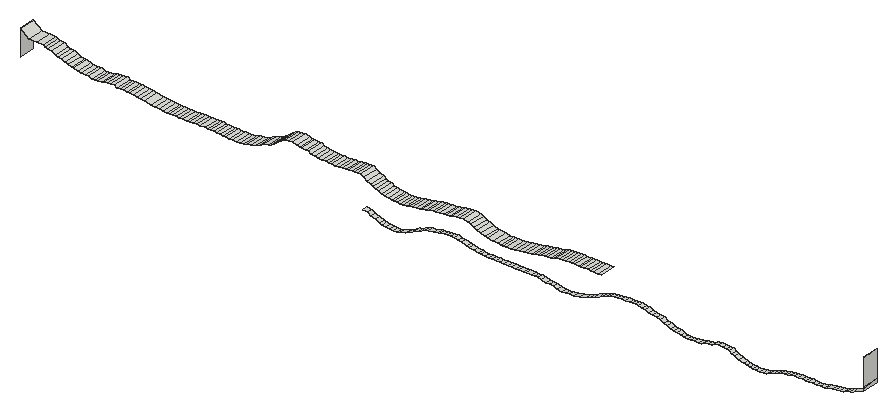
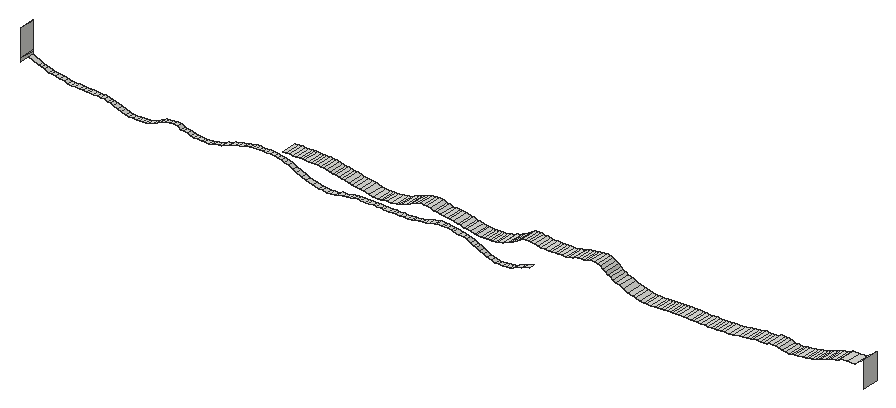
# SketchUp Ruby script. Lengths in inches.
U = 1.inch
M = Sketchup.active_model
def pt(a) = Geom::Point3d.new(a.map { |v| v * U })
def face(e, loops, mat)
  f = e.add_face(loops[0].map { |a| pt(a) })
  loops[1..].each { |l| e.add_face(l.map { |a| pt(a) }).erase! }
  f.material = f.back_material = mat if mat
  f
end
# faces: each face lists its corners as indices into pts; further lists are holes
def faces(e, pts, list, mat = nil) = list.each { |f| face(e, (f[0].is_a?(Array) ? f : [f]).map { |l| l.map { |i| pts[i] } }, mat) }
# xy, xz, yz: faces in a plane at the given z, y or x. An outline is a flat list of corners, or four numbers for a rectangle; further outlines are holes
def ring(l) = l.size == 4 ? [[l[0], l[1]], [l[2], l[1]], [l[2], l[3]], [l[0], l[3]]] : l.each_slice(2).to_a
def flat(e, list, mat, &to3) = list.each { |f| face(e, (f[0].is_a?(Array) ? f : [f]).map { |l| ring(l).map { |u, v| to3.(u, v) } }, mat) }
def xy(e, z, list, mat = nil) = flat(e, list, mat) { |x, y| [x, y, z] }
def xz(e, y, list, mat = nil) = flat(e, list, mat) { |x, z| [x, y, z] }
def yz(e, x, list, mat = nil) = flat(e, list, mat) { |y, z| [x, y, z] }
def lines(e, pts, list) = list.each { |a, b| e.add_line(pt(pts[a]), pt(pts[b])) }
# prism: a flat outline (further loops are holes) pulled along v
def prism(e, loops, v, mat = nil)
  f = face(e, loops, mat); d = Geom::Vector3d.new(v.map { |x| x * U })
  f.pushpull(f.normal.samedirection?(d) ? d.length : -d.length)
end
def box(e, o, s, mat = nil) = prism(e, [[o, [o[0] + s[0], o[1], o[2]], [o[0] + s[0], o[1] + s[1], o[2]], [o[0], o[1] + s[1], o[2]]]], [0, 0, s[2]], mat)
def at(x, y, z, deg = 0) = Geom::Transformation.translation(pt([x, y, z])) * Geom::Transformation.rotation(ORIGIN, Z_AXIS, deg.degrees)
def axes(o, x, y, z) = Geom::Transformation.new([*x, 0, *y, 0, *z, 0, *pt(o).to_a, 1])
def part(name) = M.definitions.add(name)
# library, detail: a bought-in or finely detailed component or shape, given as its bounding box
def library(name, o, s) = part(name).tap { |d| box(d.entities, o, s) }
def detail(e, o, s) = box(e.add_group.entities, o, s)
def put(e, d, t, mat = nil) = e.add_instance(d, t).tap { |i| i.material = mat if mat }
def group(e, t, mat = nil) = e.add_group.tap { |g| g.transformation = t; g.material = mat if mat }.entities
root = M.entities
xy(root,238.18,[[1254.78,2401.37,1255.46,2402.3]])
xy(root,238.62,[[1221.31,2401.37,1222.08,2402.3],[1222.08,2401.37,1222.71,2402.3],[1222.71,2401.37,1223.47,2402.3],[1223.47,2401.37,1224.09,2402.3],[1224.09,2401.37,1224.94,2402.3],
  [1224.94,2401.37,1225.58,2402.3],[1225.58,2401.37,1226.2,2402.3]])
xy(root,238.625,[[1219.89,2401.37,1220.75,2402.3]])
xy(root,238.89,[[1275.7,2401.37,1276.38,2402.3]])
xy(root,238.9,[[1277.14,2401.37,1277.76,2402.3],[1277.76,2401.37,1278.53,2402.3]])
xy(root,240.43,[[1243.98,2401.37,1244.55,2402.3]])
xy(root,241.68,[[1162.03,2401.37,1162.62,2404.3]])
xy(root,241.75,[[1164.38,2401.37,1165.25,2404.3],[1165.25,2401.37,1165.87,2404.3],[1165.87,2401.37,1166.38,2404.3]])
xy(root,243.05,[[1237.04,2401.37,1237.72,2404.3]])
xy(root,243.07,[[1235.1875,2401.37,1235.77,2404.3]])
xy(root,243.09,[[1231.875,2401.37,1232.4,2404.3],[1232.4,2401.37,1232.92,2404.3],[1232.92,2401.37,1233.58,2404.3],[1233.58,2401.37,1234.03,2404.3]])
yz(root,1131.59,[[2401.37,241.52,2404.3,246.2]])
yz(root,1285.6,[[2401.37,240.89,2401.37,241.29,2404.3,241.52,2404.3,240.89],[2401.37,241.29,2404.3,241.52,2401.37,241.52],[2401.37,241.52,2401.37,246.27,2402.0625,246.36,2404.3,246.43,2404.3,241.52],[2401.37,246.27,2401.37,246.43,2404.3,246.43,2402.0625,246.36]])
p = [[1198.39,2401.37,237.11],[1198.39,2402.3,237.11],[1199.15,2402.3,237.04],[1199.15,2401.37,237.04],[1199.84,2402.3,237.01],[1199.84,2401.37,237.01],
  [1200.45,2402.3,236.98],[1200.45,2401.37,236.98],[1201.13,2402.3,237.22],[1201.13,2401.37,237.22],[1197.7,2401.37,237.2],[1197.7,2402.3,237.2],
  [1197.17,2401.37,237.33],[1197.17,2402.3,237.33],[1201.98,2402.3,237.43],[1201.98,2401.37,237.43],[1196.5,2401.37,237.68],[1196.5,2402.3,237.68],
  [1202.6,2402.3,237.74],[1202.6,2401.37,237.74],[1265.43,2401.37,237.45],[1265.43,2402.3,237.45],[1266,2402.3,237.42],[1266,2401.37,237.42],
  [1266.73,2402.3,237.4],[1266.73,2401.37,237.4],[1267.41,2402.3,237.47],[1267.41,2401.37,237.47],[1264.24,2401.37,237.59],[1264.24,2402.3,237.59],
  [1264.84,2402.3,237.51],[1264.84,2401.37,237.51],[1268.01,2402.3,237.5625],[1268.01,2401.37,237.5625],[1263.7,2401.37,237.71],[1263.7,2402.3,237.71],
  [1268.7,2402.3,237.84],[1268.7,2401.37,237.84],[1195.5625,2401.37,237.96],[1195.5625,2402.3,237.96],[1203.3,2402.3,238.02],[1203.3,2401.37,238.02],
  [1230.44,2401.37,237.79],[1230.44,2402.3,237.79],[1231.15,2402.3,237.74],[1231.15,2401.37,237.74],[1232.02,2402.3,237.87],[1232.02,2401.37,237.87],
  [1262.87,2401.37,238],[1262.87,2402.3,238],[1229.67,2401.37,237.86],[1229.67,2402.3,237.86],[1269.38,2402.3,238.08],[1269.38,2401.37,238.08],
  [1229.04,2401.37,238.15],[1229.04,2402.3,238.15],[1232.67,2402.3,237.88],[1232.67,2401.37,237.88],[1233.79,2402.3,238.14],[1233.79,2401.37,238.14],
  [1195,2401.37,238.28],[1195,2402.3,238.28],[1203.74,2402.3,238.375],[1203.74,2401.37,238.375],[1262.16,2401.37,238.33],[1262.16,2402.3,238.33],
  [1228.27,2401.37,238.19],[1228.27,2402.3,238.19],[1235.01,2402.3,238.46],[1235.01,2401.37,238.46],[1252.76,2401.37,238.19],[1252.76,2402.3,238.19],
  [1253.58,2402.3,238.15],[1253.58,2401.37,238.15],[1254.11,2402.3,238.11],[1254.11,2401.37,238.11],[1254.78,2402.3,238.18],[1254.78,2401.37,238.18],
  [1270.07,2402.3,238.33],[1270.07,2401.37,238.33],[1227.65,2401.37,238.25],[1227.65,2402.3,238.25],[1252.1875,2401.37,238.26],[1252.1875,2402.3,238.26],
  [1255.46,2401.37,238.18],[1255.46,2402.3,238.18],[1256.14,2402.3,238.27],[1256.14,2401.37,238.27],[1194.22,2401.37,238.43],[1194.22,2402.3,238.43],
  [1226.89,2401.37,238.45],[1226.89,2402.3,238.45],[1251.62,2401.37,238.48],[1251.62,2402.3,238.48],[1256.66,2402.3,238.55],[1256.66,2401.37,238.55],
  [1261.61,2401.37,238.57],[1261.61,2402.3,238.57],[1270.6,2402.3,238.51],[1270.6,2401.37,238.51],[1204.3,2402.3,238.51],[1204.3,2401.37,238.51],
  [1204.9375,2402.3,238.76],[1204.9375,2401.37,238.76],[1226.2,2401.37,238.62],[1226.2,2402.3,238.62],[1235.76,2402.3,238.72],[1235.76,2401.37,238.72],
  [1250.96,2401.37,238.56],[1250.96,2402.3,238.56],[1257.32,2402.3,238.61],[1257.32,2401.37,238.61],[1271.17,2402.3,238.6],[1271.17,2401.37,238.6],
  [1217.13,2401.37,238.66],[1217.13,2402.3,238.66],[1217.8,2402.3,238.65],[1217.8,2401.37,238.65],[1218.58,2402.3,238.64],[1218.58,2401.37,238.64],
  [1219.2,2402.3,238.63],[1219.2,2401.37,238.63],[1219.89,2402.3,238.625],[1219.89,2401.37,238.625],[1220.75,2401.37,238.625],[1220.75,2402.3,238.625],
  [1221.31,2402.3,238.62],[1221.31,2401.37,238.62],[1250.39,2401.37,238.67],[1250.39,2402.3,238.67],[1257.91,2402.3,238.66],[1257.91,2401.37,238.66],
  [1261.11,2401.37,238.86],[1261.11,2402.3,238.86],[1271.83,2402.3,238.74],[1271.83,2401.37,238.74],[1215.29,2401.37,238.78],[1215.29,2402.3,238.78],
  [1215.77,2402.3,238.73],[1215.77,2401.37,238.73],[1216.44,2402.3,238.6875],[1216.44,2401.37,238.6875],[1236.64,2402.3,239.08],[1236.64,2401.37,239.08],
  [1249.87,2401.37,239.01],[1249.87,2402.3,239.01],[1258.48,2402.3,239.04],[1258.48,2401.37,239.04],[1272.41,2402.3,238.8],[1272.41,2401.37,238.8],
  [1205.58,2402.3,239.12],[1205.58,2401.37,239.12],[1214.41,2401.37,238.93],[1214.41,2402.3,238.93],[1272.98,2402.3,238.83],[1272.98,2401.37,238.83],
  [1273.72,2402.3,238.86],[1273.72,2401.37,238.86],[1213.64,2401.37,239.07],[1213.64,2402.3,239.07],[1260.59,2401.37,238.96],[1260.59,2402.3,238.96],
  [1274.48,2402.3,238.875],[1274.48,2401.37,238.875],[1275.02,2402.3,238.88],[1275.02,2401.37,238.88],[1275.7,2402.3,238.89],[1275.7,2401.37,238.89],
  [1276.38,2401.37,238.89],[1276.38,2402.3,238.89],[1277.14,2402.3,238.9],[1277.14,2401.37,238.9],[1278.53,2401.37,238.9],[1278.53,2402.3,238.9],
  [1279.16,2402.3,239.15],[1279.16,2401.37,239.15],[1249.1875,2401.37,239.18],[1249.1875,2402.3,239.18],[1259.22,2402.3,239.125],[1259.22,2401.37,239.125],
  [1259.9,2402.3,239.02],[1259.9,2401.37,239.02],[1206.16,2402.3,239.22],[1206.16,2401.37,239.22],[1213.09,2401.37,239.16],[1213.09,2402.3,239.16],
  [1237.43,2402.3,239.375],[1237.43,2401.37,239.375],[1207.16,2402.3,239.31],[1207.16,2401.37,239.31],[1212.24,2401.37,239.44],[1212.24,2402.3,239.44],
  [1248.5625,2401.37,239.5],[1248.5625,2402.3,239.5],[1279.93,2402.3,239.28],[1279.93,2401.37,239.28],[1207.97,2402.3,239.54],[1207.97,2401.37,239.54],
  [1280.73,2402.3,239.42],[1280.73,2401.37,239.42],[1211.57,2401.37,239.56],[1211.57,2402.3,239.56],[1238.17,2402.3,239.75],[1238.17,2401.37,239.75],
  [1281.45,2402.3,239.49],[1281.45,2401.37,239.49],[1208.46,2402.3,239.6],[1208.46,2401.37,239.6],[1247.8,2401.37,239.65],[1247.8,2402.3,239.65],
  [1282,2402.3,239.53],[1282,2401.37,239.53],[1282.6875,2402.3,239.81],[1282.6875,2401.37,239.81],[1209.08,2402.3,239.65],[1209.08,2401.37,239.65],
  [1209.67,2402.3,239.69],[1209.67,2401.37,239.69],[1210.96,2401.37,239.72],[1210.96,2402.3,239.72],[1210.23,2402.3,239.7],[1210.23,2401.37,239.7],
  [1238.82,2402.3,239.97],[1238.82,2401.37,239.97],[1247.1875,2401.37,239.8],[1247.1875,2402.3,239.8],[1246.43,2401.37,239.96],[1246.43,2402.3,239.96],
  [1283.21,2402.3,239.96],[1283.21,2401.37,239.96],[1239.44,2402.3,240.17],[1239.44,2401.37,240.17],[1245.78,2401.37,240.23],[1245.78,2402.3,240.23],
  [1283.77,2402.3,240.1],[1283.77,2401.37,240.1],[1285.6,2402.3,240.89],[1285.6,2401.37,240.89],[1240.12,2402.3,240.27],[1240.12,2401.37,240.27],
  [1245.2,2401.37,240.27],[1245.2,2402.3,240.27],[1240.8,2402.3,240.33],[1240.8,2401.37,240.33],[1241.49,2402.3,240.37],[1241.49,2401.37,240.37],
  [1244.55,2401.37,240.43],[1244.55,2402.3,240.43],[1242.18,2402.3,240.4],[1242.18,2401.37,240.4],[1242.875,2402.3,240.41],[1242.875,2401.37,240.41],
  [1243.4,2402.3,240.42],[1243.4,2401.37,240.42],[1243.98,2402.3,240.43],[1243.98,2401.37,240.43],[1168.01,2404.3,241.57],[1168.55,2404.3,241.53],
  [1168.55,2401.37,241.53],[1168.01,2401.37,241.57],[1169.17,2404.3,241.51],[1169.17,2401.37,241.51],[1169.72,2404.3,241.49],[1169.72,2401.37,241.49],
  [1170.42,2404.3,241.48],[1170.42,2401.37,241.48],[1171.08,2404.3,241.47],[1171.08,2401.37,241.47],[1171.65,2404.3,241.46],[1171.65,2401.37,241.46],
  [1172.36,2404.3,241.6],[1172.36,2401.37,241.6],[1218.73,2404.3,241.56],[1219.33,2404.3,241.51],[1219.33,2401.37,241.51],[1218.73,2401.37,241.56],
  [1219.78,2404.3,241.48],[1219.78,2401.37,241.48],[1220.3,2404.3,241.46],[1220.3,2401.37,241.46],[1221.17,2404.3,241.51],[1221.17,2401.37,241.51],
  [1221.89,2404.3,241.59],[1221.89,2401.37,241.59],[1167.4,2404.3,241.66],[1167.4,2401.37,241.66],[1173.09,2404.3,241.85],[1173.09,2401.37,241.85],
  [1216.91,2404.3,241.78],[1217.96,2404.3,241.63],[1217.96,2401.37,241.63],[1216.91,2401.37,241.78],[1222.83,2404.3,241.82],[1222.83,2401.37,241.82],
  [1158.37,2404.3,241.75],[1158.82,2404.3,241.74],[1158.82,2401.37,241.74],[1158.37,2401.37,241.75],[1159.37,2404.3,241.72],[1159.37,2401.37,241.72],
  [1160,2404.3,241.71],[1160,2401.37,241.71],[1160.63,2404.3,241.7],[1160.63,2401.37,241.7],[1161.36,2404.3,241.69],[1161.36,2401.37,241.69],
  [1162.03,2404.3,241.68],[1162.03,2401.37,241.68],[1162.62,2404.3,241.68],[1163.11,2404.3,241.67],[1163.11,2401.37,241.67],[1162.62,2401.37,241.68],
  [1163.8125,2404.3,241.74],[1163.8125,2401.37,241.74],[1164.38,2404.3,241.75],[1164.38,2401.37,241.75],[1166.38,2404.3,241.75],[1166.87,2404.3,241.67],
  [1166.87,2401.37,241.67],[1166.38,2401.37,241.75],[1156.18,2404.3,241.89],[1157,2404.3,241.83],[1157,2401.37,241.83],[1156.18,2401.37,241.89],
  [1157.6,2404.3,241.78],[1157.6,2401.37,241.78],[1173.76,2404.3,241.91],[1173.76,2401.37,241.91],[1199.39,2404.3,241.89],[1199.85,2404.3,241.85],
  [1199.85,2401.37,241.85],[1199.39,2401.37,241.89],[1200.37,2404.3,241.8125],[1200.37,2401.37,241.8125],[1200.88,2404.3,241.79],[1200.88,2401.37,241.79],
  [1201.46,2404.3,241.78],[1201.46,2401.37,241.78],[1202.13,2404.3,241.91],[1202.13,2401.37,241.91],[1216.42,2404.3,241.89],[1216.42,2401.37,241.89],
  [1223.61,2404.3,241.87],[1223.61,2401.37,241.87],[1155.41,2404.3,241.96],[1155.41,2401.37,241.96],[1174.66,2404.3,242.1],[1174.66,2401.37,242.1],
  [1198.83,2404.3,241.96],[1198.83,2401.37,241.96],[1202.6,2404.3,241.93],[1202.6,2401.37,241.93],[1203.27,2404.3,242.09],[1203.27,2401.37,242.09],
  [1215.78,2404.3,242.14],[1215.78,2401.37,242.14],[1224.375,2404.3,241.98],[1224.375,2401.37,241.98],[1154.24,2404.3,242.24],[1154.24,2401.37,242.24],
  [1198.15,2404.3,242.11],[1198.15,2401.37,242.11],[1224.99,2404.3,242.02],[1224.99,2401.37,242.02],[1225.64,2404.3,242.19],[1225.64,2401.37,242.19],
  [1175.43,2404.3,242.46],[1175.43,2401.37,242.46],[1197.55,2404.3,242.21],[1197.55,2401.37,242.21],[1204.04,2404.3,242.2],[1204.04,2401.37,242.2],
  [1215.02,2404.3,242.39],[1215.02,2401.37,242.39],[1153.57,2404.3,242.34],[1153.57,2401.37,242.34],[1197.04,2404.3,242.51],[1197.04,2401.37,242.51],
  [1204.54,2404.3,242.24],[1204.54,2401.37,242.24],[1205.15,2404.3,242.42],[1205.15,2401.37,242.42],[1226.34,2404.3,242.38],[1226.34,2401.37,242.38],
  [1152.91,2404.3,242.38],[1152.91,2401.37,242.38],[1152.25,2404.3,242.48],[1152.25,2401.37,242.48],[1205.7,2404.3,242.47],[1205.7,2401.37,242.47],
  [1214.4,2404.3,242.65],[1214.4,2401.37,242.65],[1226.83,2404.3,242.4375],[1226.83,2401.37,242.4375],[1227.35,2404.3,242.48],[1227.35,2401.37,242.48],
  [1144.07,2404.3,242.68],[1144.74,2404.3,242.51],[1144.74,2401.37,242.51],[1144.07,2401.37,242.68],[1145.26,2404.3,242.46],[1145.26,2401.37,242.46],
  [1145.8,2404.3,242.58],[1145.8,2401.37,242.58],[1151.61,2404.3,242.57],[1151.61,2401.37,242.57],[1176.13,2404.3,242.78],[1176.13,2401.37,242.78],
  [1196.45,2404.3,242.68],[1196.45,2401.37,242.68],[1206.45,2404.3,242.71],[1206.45,2401.37,242.71],[1228.01,2404.3,242.58],[1228.01,2401.37,242.58],
  [1146.43,2404.3,242.57],[1146.43,2401.37,242.57],[1147.06,2404.3,242.81],[1147.06,2401.37,242.81],[1148.83,2404.3,242.92],[1149.26,2404.3,242.625],
  [1149.26,2401.37,242.625],[1148.83,2401.37,242.92],[1149.87,2404.3,242.65],[1149.87,2401.37,242.65],[1150.42,2404.3,242.62],[1150.42,2401.37,242.62],
  [1151.05,2404.3,242.58],[1151.05,2401.37,242.58],[1213.85,2404.3,242.9375],[1213.85,2401.37,242.9375],[1228.54,2404.3,242.61],[1228.54,2401.37,242.61],
  [1229.125,2404.3,242.77],[1229.125,2401.37,242.77],[1142.72,2404.3,242.78],[1143.53,2404.3,242.73],[1143.53,2401.37,242.73],[1142.72,2401.37,242.78],
  [1195.95,2404.3,242.875],[1195.95,2401.37,242.875],[1207.09,2404.3,242.78],[1207.09,2401.37,242.78],[1141.42,2404.3,243.06],[1142.14,2404.3,242.85],
  [1142.14,2401.37,242.85],[1141.42,2401.37,243.06],[1147.63,2404.3,242.86],[1147.63,2401.37,242.86],[1176.9,2404.3,242.97],[1176.9,2401.37,242.97],
  [1207.57,2404.3,242.82],[1207.57,2401.37,242.82],[1208.26,2404.3,242.85],[1208.26,2401.37,242.85],[1229.58,2404.3,242.95],[1229.58,2401.37,242.95],
  [1148.19,2404.3,242.89],[1148.19,2401.37,242.89],[1195.56,2404.3,243.09],[1195.56,2401.37,243.09],[1208.96,2404.3,242.87],[1208.96,2401.37,242.87],
  [1209.51,2404.3,243.02],[1209.51,2401.37,243.02],[1213.28,2404.3,243.14],[1213.28,2401.37,243.14],[1177.43,2404.3,243.23],[1177.43,2401.37,243.23],
  [1210.13,2404.3,243.05],[1210.13,2401.37,243.05],[1230.14,2404.3,243.01],[1230.14,2401.37,243.01],[1230.65,2404.3,243.05],[1230.65,2401.37,243.05],
  [1231.22,2404.3,243.08],[1231.22,2401.37,243.08],[1140.35,2404.3,243.3],[1140.9375,2404.3,243.14],[1140.9375,2401.37,243.14],[1140.35,2401.37,243.3],
  [1194.95,2404.3,243.43],[1194.95,2401.37,243.43],[1210.68,2404.3,243.29],[1210.68,2401.37,243.29],[1212.51,2404.3,243.42],[1212.51,2401.37,243.42],
  [1231.875,2404.3,243.09],[1231.875,2401.37,243.09],[1234.03,2404.3,243.09],[1234.6,2404.3,243.08],[1234.6,2401.37,243.08],[1234.03,2401.37,243.09],
  [1235.1875,2404.3,243.07],[1235.1875,2401.37,243.07],[1235.77,2404.3,243.07],[1236.43,2404.3,243.0625],[1236.43,2401.37,243.0625],[1235.77,2401.37,243.07],
  [1237.04,2404.3,243.05],[1237.04,2401.37,243.05],[1177.83,2404.3,243.48],[1177.83,2401.37,243.48],[1139.71,2404.3,243.48],[1139.71,2401.37,243.48],
  [1211.36,2404.3,243.35],[1211.36,2401.37,243.35],[1194.41,2404.3,243.8],[1194.41,2401.37,243.8],[1211.91,2404.3,243.39],[1211.91,2401.37,243.39],
  [1139.19,2404.3,243.79],[1139.19,2401.37,243.79],[1178.35,2404.3,243.72],[1178.35,2401.37,243.72],[1178.6875,2404.3,244.12],[1178.6875,2401.37,244.12],
  [1138.53,2404.3,243.95],[1138.53,2401.37,243.95],[1193.81,2404.3,244.18],[1193.81,2401.37,244.18],[1138.01,2404.3,244.11],[1138.01,2401.37,244.11],
  [1186.63,2404.3,243.99],[1187.35,2404.3,243.95],[1187.35,2401.37,243.95],[1186.63,2401.37,243.99],[1187.85,2404.3,243.93],[1187.85,2401.37,243.93],
  [1188.54,2404.3,243.91],[1188.54,2401.37,243.91],[1189.11,2404.3,243.89],[1189.11,2401.37,243.89],[1189.81,2404.3,243.88],[1189.81,2401.37,243.88],
  [1190.46,2404.3,243.94],[1190.46,2401.37,243.94],[1191.1,2404.3,243.95],[1191.1,2401.37,243.95],[1191.66,2404.3,244.1],[1191.66,2401.37,244.1],
  [1185.45,2404.3,244.11],[1186.01,2404.3,244.04],[1186.01,2401.37,244.04],[1185.45,2401.37,244.11],[1137.34,2404.3,244.41],[1137.34,2401.37,244.41],
  [1179.16,2404.3,244.39],[1179.16,2401.37,244.39],[1184.7,2404.3,244.25],[1184.7,2401.37,244.25],[1192.29,2404.3,244.13],[1192.29,2401.37,244.13],
  [1192.77,2404.3,244.15],[1192.77,2401.37,244.15],[1193.29,2404.3,244.17],[1193.29,2401.37,244.17],[1184.24,2404.3,244.51],[1184.24,2401.37,244.51],
  [1136.58,2404.3,244.54],[1136.58,2401.37,244.54],[1179.64,2404.3,244.73],[1179.64,2401.37,244.73],[1136.02,2404.3,244.61],[1136.02,2401.37,244.61],
  [1183.09,2404.3,244.67],[1183.7,2404.3,244.55],[1183.7,2401.37,244.55],[1183.09,2401.37,244.67],[1135.8,2404.3,244.92],[1135.8,2401.37,244.92],
  [1180.125,2404.3,244.87],[1180.125,2401.37,244.87],[1182.04,2404.3,244.81],[1182.61,2404.3,244.7],[1182.61,2401.37,244.7],[1182.04,2401.37,244.81],
  [1181.39,2404.3,245.01],[1181.39,2401.37,245.01],[1133.16,2404.3,244.96],[1134.55,2404.3,244.9375],[1134.55,2401.37,244.9375],[1133.16,2401.37,244.96],
  [1180.71,2404.3,244.95],[1180.71,2401.37,244.95],[1131.59,2404.3,246.2],[1131.59,2401.37,246.2]]
faces(root,p,[[0,1,2,3],[3,2,4,5],[5,4,6,7],[7,6,8,9],[10,11,1,0],[12,13,11,10],[9,8,14,15],[16,17,13,12],
  [15,14,18,19],[20,21,22,23],[23,22,24,25],[25,24,26,27],[28,29,30,31],[31,30,21,20],[27,26,32,33],[34,35,29,28],
  [33,32,36,37],[38,39,17,16],[19,18,40,41],[42,43,44,45],[45,44,46,47],[48,49,35,34],[50,51,43,42],[37,36,52,53],
  [54,55,51,50],[47,46,56,57],[57,56,58,59],[60,61,39,38],[41,40,62,63],[64,65,49,48],[66,67,55,54],[59,58,68,69],
  [70,71,72,73],[73,72,74,75],[75,74,76,77],[53,52,78,79],[80,81,67,66],[82,83,71,70],[84,85,86,87],[88,89,61,60],
  [90,91,81,80],[92,93,83,82],[87,86,94,95],[96,97,65,64],[79,78,98,99],[63,62,100,101],[101,100,102,103],[104,105,91,90],
  [69,68,106,107],[108,109,93,92],[95,94,110,111],[99,98,112,113],[114,115,116,117],[117,116,118,119],[119,118,120,121],[121,120,122,123],
  [124,125,126,127],[128,129,109,108],[111,110,130,131],[132,133,97,96],[113,112,134,135],[136,137,138,139],[139,138,140,141],[141,140,115,114],
  [107,106,142,143],[144,145,129,128],[131,130,146,147],[135,134,148,149],[103,102,150,151],[152,153,137,136],[149,148,154,155],[155,154,156,157],
  [158,159,153,152],[160,161,133,132],[157,156,162,163],[163,162,164,165],[165,164,166,167],[168,169,170,171],[172,173,174,175],[176,177,145,144],
  [147,146,178,179],[179,178,180,181],[181,180,161,160],[151,150,182,183],[184,185,159,158],[143,142,186,187],[183,182,188,189],[190,191,185,184],
  [192,193,177,176],[175,174,194,195],[189,188,196,197],[195,194,198,199],[200,201,191,190],[187,186,202,203],[199,198,204,205],[197,196,206,207],
  [208,209,193,192],[205,204,210,211],[211,210,212,213],[207,206,214,215],[215,214,216,217],[218,219,201,200],[217,216,220,221],[221,220,219,218],
  [203,202,222,223],[224,225,209,208],[226,227,225,224],[213,212,228,229],[223,222,230,231],[232,233,227,226],[229,228,234,235],[235,234,236,237],
  [231,230,238,239],[240,241,233,232],[239,238,242,243],[243,242,244,245],[246,247,241,240],[245,244,248,249],[249,248,250,251],[251,250,252,253],
  [253,252,254,255],[256,257,258,259],[257,260,261,258],[260,262,263,261],[262,264,265,263],[264,266,267,265],[266,268,269,267],[268,270,271,269],
  [272,273,274,275],[273,276,277,274],[276,278,279,277],[278,280,281,279],[280,282,283,281],[284,256,259,285],[270,286,287,271],[288,289,290,291],
  [289,272,275,290],[282,292,293,283],[294,295,296,297],[295,298,299,296],[298,300,301,299],[300,302,303,301],[302,304,305,303],[304,306,307,305],
  [308,309,310,311],[309,312,313,310],[312,314,315,313],[316,317,318,319],[317,284,285,318],[320,321,322,323],[321,324,325,322],[324,294,297,325],
  [286,326,327,287],[328,329,330,331],[329,332,333,330],[332,334,335,333],[334,336,337,335],[336,338,339,337],[340,288,291,341],[292,342,343,293],
  [344,320,323,345],[326,346,347,327],[348,328,331,349],[338,350,351,339],[350,352,353,351],[354,340,341,355],[342,356,357,343],[358,344,345,359],
  [360,348,349,361],[356,362,363,357],[362,364,365,363],[346,366,367,347],[368,360,361,369],[352,370,371,353],[372,354,355,373],[374,358,359,375],
  [376,368,369,377],[370,378,379,371],[378,380,381,379],[364,382,383,365],[384,374,375,385],[386,384,385,387],[380,388,389,381],[390,372,373,391],
  [382,392,393,383],[392,394,395,393],[396,397,398,399],[397,400,401,398],[400,402,403,401],[404,386,387,405],[366,406,407,367],[408,376,377,409],
  [388,410,411,389],[394,412,413,395],[402,414,415,403],[414,416,417,415],[418,419,420,421],[419,422,423,420],[422,424,425,423],[424,426,427,425],
  [426,404,405,427],[428,390,391,429],[412,430,431,413],[430,432,433,431],[434,435,436,437],[435,396,399,436],[438,408,409,439],[410,440,441,411],
  [442,443,444,445],[443,434,437,444],[416,446,447,417],[406,448,449,407],[440,450,451,441],[450,452,453,451],[432,454,455,433],[446,456,457,447],
  [456,418,421,457],[458,438,439,459],[452,460,461,453],[460,462,463,461],[464,428,429,465],[448,466,467,449],[462,468,469,463],[454,470,471,455],
  [470,472,473,471],[472,474,475,473],[476,477,478,479],[477,442,445,478],[480,458,459,481],[468,482,483,469],[484,464,465,485],[474,486,487,475],
  [488,489,490,491],[489,492,493,490],[494,495,496,497],[495,498,499,496],[466,500,501,467],[502,476,479,503],[482,504,505,483],[506,480,481,507],
  [504,508,509,505],[508,484,485,509],[510,502,503,511],[500,512,513,501],[512,514,515,513],[516,510,511,517],[518,506,507,519],[520,516,517,521],
  [522,523,524,525],[523,526,527,524],[526,528,529,527],[528,530,531,529],[530,532,533,531],[532,534,535,533],[534,536,537,535],[536,538,539,537],
  [540,541,542,543],[541,522,525,542],[544,520,521,545],[514,546,547,515],[548,540,543,549],[538,550,551,539],[550,552,553,551],[552,554,555,553],
  [554,518,519,555],[556,548,549,557],[558,544,545,559],[546,560,561,547],[562,558,559,563],[564,565,566,567],[565,556,557,566],[568,562,563,569],
  [560,570,571,561],[572,573,574,575],[573,564,567,574],[576,572,575,577],[578,579,580,581],[579,568,569,580],[570,582,583,571],[582,576,577,583],
  [584,578,581,585]])
